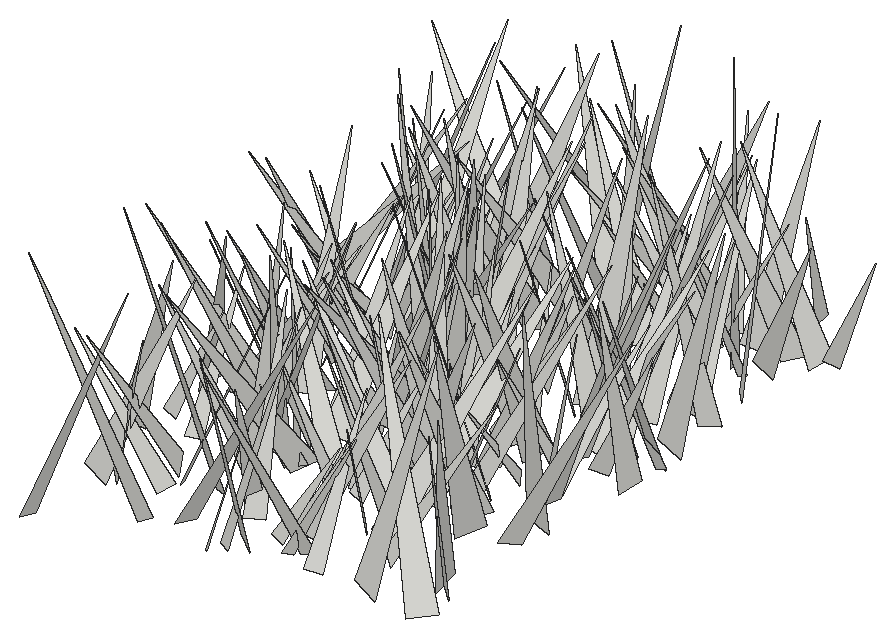
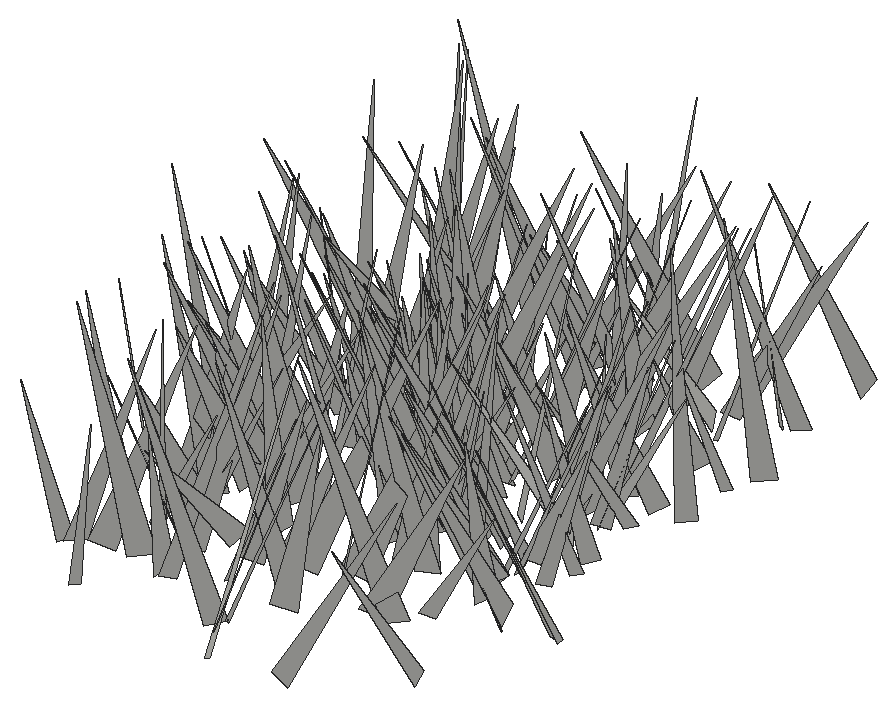
# SketchUp Ruby script. Lengths in inches.
U = 1.inch
M = Sketchup.active_model
def pt(a) = Geom::Point3d.new(a.map { |v| v * U })
def face(e, loops, mat)
  f = e.add_face(loops[0].map { |a| pt(a) })
  loops[1..].each { |l| e.add_face(l.map { |a| pt(a) }).erase! }
  f.material = f.back_material = mat if mat
  f
end
# faces: each face lists its corners as indices into pts; further lists are holes
def faces(e, pts, list, mat = nil) = list.each { |f| face(e, (f[0].is_a?(Array) ? f : [f]).map { |l| l.map { |i| pts[i] } }, mat) }
# xy, xz, yz: faces in a plane at the given z, y or x. An outline is a flat list of corners, or four numbers for a rectangle; further outlines are holes
def ring(l) = l.size == 4 ? [[l[0], l[1]], [l[2], l[1]], [l[2], l[3]], [l[0], l[3]]] : l.each_slice(2).to_a
def flat(e, list, mat, &to3) = list.each { |f| face(e, (f[0].is_a?(Array) ? f : [f]).map { |l| ring(l).map { |u, v| to3.(u, v) } }, mat) }
def xy(e, z, list, mat = nil) = flat(e, list, mat) { |x, y| [x, y, z] }
def xz(e, y, list, mat = nil) = flat(e, list, mat) { |x, z| [x, y, z] }
def yz(e, x, list, mat = nil) = flat(e, list, mat) { |y, z| [x, y, z] }
def lines(e, pts, list) = list.each { |a, b| e.add_line(pt(pts[a]), pt(pts[b])) }
# prism: a flat outline (further loops are holes) pulled along v
def prism(e, loops, v, mat = nil)
  f = face(e, loops, mat); d = Geom::Vector3d.new(v.map { |x| x * U })
  f.pushpull(f.normal.samedirection?(d) ? d.length : -d.length)
end
def box(e, o, s, mat = nil) = prism(e, [[o, [o[0] + s[0], o[1], o[2]], [o[0] + s[0], o[1] + s[1], o[2]], [o[0], o[1] + s[1], o[2]]]], [0, 0, s[2]], mat)
def at(x, y, z, deg = 0) = Geom::Transformation.translation(pt([x, y, z])) * Geom::Transformation.rotation(ORIGIN, Z_AXIS, deg.degrees)
def axes(o, x, y, z) = Geom::Transformation.new([*x, 0, *y, 0, *z, 0, *pt(o).to_a, 1])
def part(name) = M.definitions.add(name)
# library, detail: a bought-in or finely detailed component or shape, given as its bounding box
def library(name, o, s) = part(name).tap { |d| box(d.entities, o, s) }
def detail(e, o, s) = box(e.add_group.entities, o, s)
def put(e, d, t, mat = nil) = e.add_instance(d, t).tap { |i| i.material = mat if mat }
def group(e, t, mat = nil) = e.add_group.tap { |g| g.transformation = t; g.material = mat if mat }.entities
root = M.entities
c1 = part("fur_instance\#9")
p = [[0.8125,0,1.79],[0.67,-0.02,1.48],[0,-0.11,0],[0,0.11,0]]
faces(c1.entities,p,[[0,1,2,3]])
put(root,c1,axes([528.57,193.91,-21.66],[-2.74524,3.88345,0.46197],[3.73915,2.44095,1.70042],[-1.14601,-1.33847,4.4414]))
put(root,c1,axes([528.73,186.81,-21.66],[-3.23089,-3.2407,0.20186],[-3.09319,2.98531,-1.58167],[-0.98745,1.25194,4.29408]))
put(root,c1,axes([525.39,207.13,-21.66],[4.79921,1.03907,0.41248],[0.79797,-4.45725,1.94381],[-0.78297,1.82633,4.50929]))
put(root,c1,axes([522.77,199.48,-21.66],[5.32286,5.30667,0.20638],[4.93366,-4.8331,-2.97258],[1.96528,-2.23975,6.90343]))
put(root,c1,axes([526.5,195.48,-21.66],[-6.90134,-2.30385,2.57209],[-0.73953,6.60101,3.92832],[3.37291,-3.26662,6.12409]))
put(root,c1,axes([522.13,199.56,-21.66],[4.7067,5.43888,0.18038],[4.50837,-3.76361,-4.15655],[3.04771,-2.83211,5.87006]))
put(root,c1,axes([529.1875,201.72,-21.66],[-2.95637,3.32548,0.26078],[3.10336,2.61427,1.84435],[-1.22309,-1.40488,4.04936]))
put(root,c1,axes([524.52,179.79,-21.66],[2.49015,-6.48815,0.76577],[-6.33726,-2.19962,1.97082],[1.58797,1.39602,6.66429]))
put(root,c1,axes([525.36,181.79,-21.66],[0.91676,-3.52562,1.5814],[-3.59518,-0.18259,1.67709],[1.41617,1.81877,3.23385]))
put(root,c1,axes([526.02,199.09,-21.66],[6.68377,2.4417,1.0502],[1.89436,-6.36953,2.75283],[-1.86446,2.28139,6.56175]))
put(root,c1,axes([527.9,198.42,-21.66],[-5.38629,2.97439,0.98855],[2.72826,5.41671,-1.43257],[1.54299,0.80541,5.98388]))
put(root,c1,axes([528.33,195.32,-21.66],[-6.95908,-3.88864,0.42907],[-3.38575,6.42493,3.31533],[1.96017,-2.70799,7.24975]))
put(root,c1,axes([531.37,172.26,-21.66],[-3.36679,-6.63148,1.92496],[-6.20382,1.96447,-4.08298],[-3.03226,3.34389,6.21619]))
put(root,c1,axes([524.98,185.625,-21.66],[6.92696,-1.79403,0.01467],[-1.72828,-6.68834,-1.86567],[-0.48147,-1.80253,6.90801]))
put(root,c1,axes([525.2,200.62,-21.66],[3.3764,2.66955,0.1135],[2.47122,-3.05035,-1.76859],[1.01611,-1.452,3.92412]))
put(root,c1,axes([529.14,185.84,-21.66],[-7.53778,-2.79862,0.78068],[-2.32716,7.11502,3.03655],[1.73954,-2.60846,7.44512]))
put(root,c1,axes([528.0625,189.09,-21.66],[-4.13321,-3.41194,0.20507],[-3.07913,3.85633,2.10107],[1.48403,-1.5014,4.93054]))
put(root,c1,axes([531.46,203.31,-21.66],[-4.54084,5.90887,0.08971],[5.53212,4.21055,2.68494],[-2.07809,-1.7025,6.95162]))
put(root,c1,axes([528.06,188.81,-21.66],[2.83348,-4.00549,0.52306],[-3.76222,-2.8494,-1.43972],[-1.47079,-0.42795,4.69039]))
put(root,c1,axes([527.96,180.57,-21.66],[-3.50119,3.09472,0.56001],[2.74674,3.41714,-1.71109],[1.53177,0.94611,4.34831]))
put(root,c1,axes([526.14,192.05,-21.66],[2.61538,-3.98544,0.72253],[-3.93735,-2.29982,1.56655],[0.95028,1.43982,4.50221]))
put(root,c1,axes([526.34,168.91,-21.66],[6.82155,0.82248,0.97272],[0.53436,-6.65794,1.88216],[-1.15634,1.77527,6.60814]))
put(root,c1,axes([530.17,175.51,-21.66],[-4.08347,2.98679,1.40676],[3.27171,3.36098,2.36101],[-0.44252,-2.71247,4.47451]))
put(root,c1,axes([528.46,194.88,-21.66],[-4.47086,-3.62986,0.22446],[-3.11938,4.01034,2.72058],[1.8697,-1.98902,5.07572]))
put(root,c1,axes([525.89,193.55,-21.66],[1.52671,4.77623,1.67607],[4.63081,-0.61106,-2.47682],[2.04382,-2.18327,4.35989]))
put(root,c1,axes([528.67,191.63,-21.66],[3.08843,-3.08617,0.55459],[-2.71507,-3.02147,-1.69397],[-1.56857,-0.84658,4.0241]))
put(root,c1,axes([528.7,196.97,-21.66],[-6.04626,5.73242,0.3376],[5.11125,5.59588,-3.47751],[2.61721,2.31459,7.57131]))
put(root,c1,axes([528.83,195.85,-21.66],[-4.31312,-2.31019,0.44376],[-1.59331,3.55068,2.99849],[1.73068,-2.4885,3.8664]))
put(root,c1,axes([530.14,188.78,-21.66],[-0.06223,-5.95217,0.13196],[-5.73579,0.02457,-1.59678],[-1.59576,0.14382,5.73432]))
put(root,c1,axes([527.31,174.9,-21.66],[3.73633,3.15118,1.53756],[3.50493,-3.41917,-1.50964],[-0.09758,-2.15258,4.64878]))
put(root,c1,axes([530.96,211.68,-21.66],[-0.84326,-5.89202,0.02664],[-5.53518,0.78295,-2.04363],[-2.01949,0.3143,5.59022]))
put(root,c1,axes([529.37,187.77,-21.66],[-5.90287,3.96424,1.22936],[3.5461,5.92766,-2.08769],[2.15678,1.10365,6.7971]))
put(root,c1,axes([526.81,187.87,-21.66],[0.32449,4.79651,0.65441],[4.29347,0.01783,-2.25961],[2.23626,-0.73022,4.24334]))
put(root,c1,axes([529.14,177.98,-21.66],[-5.60645,-3.595,0.79099],[-2.74257,5.04084,3.47133],[2.4552,-2.57833,5.68385]))
put(root,c1,axes([528.8,193.94,-21.66],[3.99187,0.97882,1.10255],[0.50795,-3.90054,1.62373],[-1.38409,1.39155,3.77579]))
put(root,c1,axes([528.23,190.94,-21.66],[6.17595,4.1917,0.11311],[3.92557,-5.85042,2.46738],[-1.47413,1.98185,7.04448]))
put(root,c1,axes([526.33,174.45,-21.66],[1.93796,6.92662,2.2466],[6.80944,-0.90011,-3.09877],[2.58009,-2.82714,6.49087]))
put(root,c1,axes([532.58,176.99,-21.66],[-5.1387,-6.17044,1.38685],[-6.22365,4.61615,-2.52214],[-1.12419,2.64967,7.62361]))
put(root,c1,axes([528.51,196.39,-21.66],[4.2696,-0.12633,0.87704],[-0.45536,-4.01534,1.6384],[-0.76014,1.6958,3.94476]))
put(root,c1,axes([526.8,185.56,-21.66],[4.24231,-3.44067,0.07958],[-3.18347,-3.87509,2.16585],[1.3077,1.72835,5.01442]))
put(root,c1,axes([531.67,194.64,-21.66],[3.01287,6.59159,3.14785],[6.68601,-3.85992,1.68335],[-2.94198,-2.02171,7.04931]))
put(root,c1,axes([528.9,185.46,-21.66],[-0.2633,5.21725,2.01289],[5.21535,0.95622,-1.79623],[2.01778,-1.79073,4.90536]))
put(root,c1,axes([533.96,181.52,-21.66],[-0.88156,-7.55851,1.51866],[-6.98391,0.13553,-3.37952],[-3.26533,1.75074,6.81814]))
put(root,c1,axes([532.01,183.98,-21.66],[2.11114,4.26728,1.69749],[4.08085,-2.60007,1.46097],[-2.10662,-0.76029,4.53125]))
put(root,c1,axes([532.69,179.58,-21.66],[-6.28485,-0.79991,0.77187],[-0.56549,6.11624,1.73401],[0.95701,-1.63912,6.09364]))
put(root,c1,axes([532.57,184.47,-21.66],[-6.5639,-4.29471,0.69968],[-4.06333,6.50273,1.7952],[1.55674,-1.13527,7.63588]))
put(root,c1,axes([533.91,193.32,-21.66],[-6.55777,-1.69063,0.96933],[-1.94723,5.82112,-3.02077],[0.07829,3.17151,6.06115]))
put(root,c1,axes([530.46,176.52,-21.66],[5.39727,3.08007,0.18691],[2.81936,-5.07536,2.22356],[-1.25418,1.84558,5.80286]))
put(root,c1,axes([531.86,190.75,-21.66],[-4.79038,-5.44103,1.36632],[-5.2062,4.98101,1.5825],[2.08977,-0.06337,7.07448]))
put(root,c1,axes([534.72,195.49,-21.66],[-3.87014,-4.65436,0.40491],[-4.4497,3.51193,-2.16136],[-1.42379,1.67578,5.65416]))
put(root,c1,axes([532.56,179.71,-21.66],[-6.83852,1.49302,2.47832],[0.97247,7.17644,-1.63995],[2.72497,1.18576,6.80477]))
put(root,c1,axes([531.94,193.09,-21.66],[6.07778,0.82962,2.17123],[-0.33597,-5.70106,3.1188],[-2.29992,3.02515,5.28212]))
put(root,c1,axes([531.69,194.95,-21.66],[4.95008,1.27612,1.12304],[0.89586,-4.89693,1.61571],[-1.4447,1.33589,4.84988]))
put(root,c1,axes([530.04,203.27,-21.66],[-0.29437,7.39176,2.68978],[7.28817,1.26884,-2.68928],[2.95898,-2.3899,6.89148]))
put(root,c1,axes([535.32,190.75,-21.66],[0.70112,8.01126,1.73468],[7.49163,-1.33281,3.12731],[-3.32639,-1.31314,7.4089]))
put(root,c1,axes([534.32,181.81,-21.66],[4.16443,-6.48584,0.7003],[-5.50995,-3.94185,-3.74183],[-3.49241,-1.51483,6.7385]))
put(root,c1,axes([534.71,200.68,-21.66],[1.87232,-8.06563,0.81969],[-7.60481,-2.03883,-2.69107],[-2.80947,0.14362,7.83059]))
put(root,c1,axes([534.64,187.95,-21.66],[-6.99156,-3.62516,0.34789],[-3.32905,6.6672,2.57109],[1.47657,-2.13338,7.444]))
put(root,c1,axes([532.94,186.05,-21.66],[-4.70627,4.28235,1.06672],[3.70191,4.67966,-2.45399],[2.40255,1.178,5.87073]))
put(root,c1,axes([531.13,192.5625,-21.66],[8.13391,1.72844,0.70897],[1.41113,-7.75982,2.72846],[-1.22428,2.53935,7.85515]))
put(root,c1,axes([533.78,197.67,-21.66],[-6.33507,2.2676,3.27677],[3.13305,6.63723,1.4641],[2.46237,-2.61105,6.56746]))
put(root,c1,axes([535.47,205.73,-21.66],[-2.86561,6.0597,1.12131],[6.09085,2.59686,1.53195],[-0.93747,-1.65086,6.5257]))
put(root,c1,axes([533.78,203.43,-21.66],[-6.24986,-4.52728,1.84324],[-4.17742,6.50052,1.80193],[2.5383,-0.44892,7.504]))
put(root,c1,axes([534.28,200.32,-21.66],[1.52611,3.71718,0.33458],[3.41655,-1.5369,1.49113],[-1.50217,0.28087,3.73135]))
put(root,c1,axes([532.07,198.11,-21.66],[0.54119,7.40359,2.44886],[7.61955,0.0202,-1.74498],[1.65906,-2.50787,7.21533]))
put(root,c1,axes([535.94,188.21,-21.66],[-4.58905,2.11277,0.48874],[2.15665,4.32669,1.54618],[-0.22698,-1.60562,4.80963]))
put(root,c1,axes([532.86,181.7,-21.66],[-0.95701,-7.3765,1.52863],[-7.35851,1.24531,1.40248],[1.61303,1.30453,7.30491]))
put(root,c1,axes([532.6,193.82,-21.66],[4.39475,-2.24157,1.41228],[-2.61052,-4.13054,1.56743],[-0.4521,2.06082,4.67778]))
put(root,c1,axes([532.31,197.92,-21.66],[1.32188,-7.44707,0.58602],[-7.30684,-1.16527,1.67389],[1.55318,0.85612,7.37593]))
put(root,c1,axes([536.4,195.35,-21.66],[1.94153,-7.03493,2.68991],[-6.84514,-2.80689,-2.40016],[-3.14163,1.7682,6.89195]))
put(root,c1,axes([536.97,191.21,-21.66],[-4.91979,-5.33902,1.78444],[-5.59743,4.38767,-2.30455],[-0.5985,2.85253,6.88466]))
put(root,c1,axes([536.98,181.16,-21.66],[-3.95209,5.35159,0.47213],[5.26841,3.74586,1.6413],[-1.05182,-1.34553,6.44707]))
put(root,c1,axes([532.88,179.36,-21.66],[7.43701,2.08557,1.03262],[1.85087,-7.39668,1.60887],[-1.41074,1.29018,7.55449]))
put(root,c1,axes([537.23,208.98,-21.66],[-6.20853,-2.44848,0.56631],[-2.51301,6.03462,-1.45936],[-0.02325,1.56521,6.51238]))
put(root,c1,axes([533.54,185.23,-21.66],[-2.62249,6.7547,0.84995],[6.3246,2.75431,-2.37468],[2.5195,0.11678,6.84575]))
put(root,c1,axes([535.32,196.39,-21.66],[5.43527,-3.00495,4.38513],[-4.48513,-5.95873,1.47596],[-2.85354,3.64214,6.0327]))
put(root,c1,axes([535.67,175.88,-21.66],[-5.09281,3.29268,0.78292],[3.01884,5.05892,-1.63872],[1.53013,0.9783,5.83893]))
put(root,c1,axes([535.88,189.28,-21.66],[2.95419,-3.46444,1.08183],[-2.95275,-3.10527,-1.88109],[-2.11044,-0.50488,4.14621]))
put(root,c1,axes([536.98,180.97,-21.66],[-0.30638,-3.92044,1.36874],[-3.76361,-0.31774,-1.75256],[-1.75458,1.36615,3.52026]))
put(root,c1,axes([537.61,203.42,-21.66],[-2.28095,-6.51713,0.89519],[-6.46928,2.05047,-1.55597],[-1.19279,1.34151,6.72716]))
put(root,c1,axes([536.82,191.13,-21.66],[-6.72767,0.28008,1.7782],[-0.11729,6.79671,-1.51427],[1.7963,1.49276,6.56102]))
put(root,c1,axes([534.35,189.71,-21.66],[0.16131,6.95669,2.04491],[7.08472,0.28432,-1.5261],[1.54396,-2.03146,6.78915]))
put(root,c1,axes([535.84,171.74,-21.66],[2.63979,2.66437,0.28601],[2.37928,-2.51517,1.47039],[-1.23275,0.85099,3.4504]))
put(root,c1,axes([537.33,201.82,-21.66],[4.76692,-6.38187,0.99404],[-5.33821,-4.5884,-3.85875],[-3.63592,-1.6304,6.96863]))
put(root,c1,axes([536.58,189.67,-21.66],[4.8815,3.3845,2.02519],[2.72156,-5.22275,2.16824],[-2.85471,0.80828,5.53015]))
put(root,c1,axes([535.125,176.72,-21.66],[4.67947,-2.49587,0.44393],[-2.29207,-4.56374,-1.49753],[-1.08298,-1.12554,5.08765]))
put(root,c1,axes([535.3,212.25,-21.66],[-5.2335,-6.40482,0.23356],[-5.52847,4.66397,4.0186],[3.24225,-2.38569,7.22925]))
put(root,c1,axes([533.09,173.48,-21.66],[7.82793,-0.68601,0.13891],[-0.69946,-7.6099,1.83483],[0.02566,1.8399,7.64072]))
put(root,c1,axes([534.08,194.3125,-21.66],[2.99312,-6.69994,0.30324],[-6.59145,-2.87731,1.48788],[1.23852,0.87852,7.18569]))
put(root,c1,axes([534.7,188.22,-21.66],[1.84734,5.85191,0.92453],[5.8229,-1.61485,-1.41361],[1.09242,-1.28828,5.97153]))
put(root,c1,axes([534.1,196.99,-21.66],[3.571,6.90444,0.98118],[6.89309,-3.32732,-1.67343],[1.05801,-1.62595,7.59098]))
put(root,c1,axes([536.84,208.65,-21.66],[-5.34969,-3.46152,0.37635],[-2.75195,4.62606,3.43064],[2.1332,-2.713,5.36954]))
put(root,c1,axes([533.3125,192,-21.66],[6.82569,-2.14516,0.01525],[-2.06759,-6.56497,1.95405],[0.57187,1.86856,6.88284]))
put(root,c1,axes([537.81,190.9,-21.66],[-6.09704,1.94582,1.05535],[1.61207,6.02238,-1.79053],[1.51697,1.42075,6.14444]))
put(root,c1,axes([536.34,172.56,-21.66],[4.01654,5.38759,0.39242],[5.219,-3.99648,1.45013],[-1.3936,0.56102,6.56169]))
put(root,c1,axes([538.27,187.49,-21.66],[-6.12572,-2.31991,2.2614],[-2.97153,5.95041,-1.94497],[1.2907,2.68904,6.25488]))
put(root,c1,axes([536.48,204.04,-21.66],[-7.17026,0.40545,3.85637],[-0.86926,7.73252,-2.42922],[3.77894,2.54801,6.75839]))
put(root,c1,axes([537.85,188.75,-21.66],[5.96387,-5.74764,0.45925],[-4.68382,-5.21453,-4.43673],[-3.36276,-2.93042,6.99418]))
put(root,c1,axes([536.92,173.59,-21.66],[-3.51133,-6.12863,1.17286],[-5.90116,3.69891,1.66117],[2.0278,0.152,6.86513]))
put(root,c1,axes([539.97,202.88,-21.66],[-3.49983,5.63032,0.78088],[5.54982,3.18646,1.89866],[-1.22869,-1.64469,6.35172]))
put(root,c1,axes([534.82,193.79,-21.66],[4.52009,6.67395,0.30614],[6.59904,-4.40227,-1.46264],[1.04307,-1.07006,7.92676]))
put(root,c1,axes([535.83,191.75,-21.66],[2.29516,-7.21123,1.1617],[-7.23425,-2.07612,1.40519],[1.00849,1.5189,7.43607]))
put(root,c1,axes([540.28,174.66,-21.66],[-1.24481,-6.10899,0.55091],[-5.80958,0.99391,-2.10566],[-1.96776,0.93016,5.86818]))
put(root,c1,axes([538.4,185.97,-21.66],[3.46655,5.88623,0.70358],[5.62008,-3.5225,1.77941],[-1.8861,0.32244,6.59533]))
put(root,c1,axes([535.91,191.65,-21.66],[0.28527,8.21503,1.11931],[7.94931,0.04717,-2.37217],[2.35543,-1.15413,7.87026]))
put(root,c1,axes([537.84,181.71,-21.66],[4.12915,-1.39251,2.24683],[-2.1688,-4.1671,1.40312],[-1.51116,2.17563,4.12556]))
put(root,c1,axes([541.44,180.73,-21.66],[-6.06762,4.08752,0.30456],[4.00596,5.79855,1.98636],[-0.86766,-1.81261,7.04117]))
put(root,c1,axes([535.37,187.67,-21.66],[3.43501,-7.39782,1.03394],[-7.28345,-3.06455,2.27067],[1.65774,1.86463,7.83397]))
put(root,c1,axes([538.56,189.65,-21.66],[6.05789,3.57549,2.196],[3.19122,-6.43003,1.66595],[-2.72445,0.41853,6.83424]))
put(root,c1,axes([539.65,182.47,-21.66],[-5.8383,-2.13052,1.19785],[-1.77007,5.82456,1.73238],[1.68547,-1.263,5.96857]))
put(root,c1,axes([538.72,188.98,-21.66],[3.46816,-3.92613,0.03464],[-3.68547,-3.27126,-1.77763],[-1.35388,-1.15247,4.92774]))
put(root,c1,axes([535.99,187.38,-21.66],[7.97506,1.59703,0.67128],[1.71117,-7.75527,-1.87893],[-0.27022,-1.97686,7.91339]))
put(root,c1,axes([539.58,205.28,-21.66],[-4.13984,-2.04423,0.54277],[-1.65039,3.86825,1.98107],[1.32277,-1.57147,4.17043]))
put(root,c1,axes([540.73,184.64,-21.66],[-0.59735,8.07244,1.41711],[8.08686,0.34954,1.4177],[-1.33238,-1.49761,7.96939]))
put(root,c1,axes([541.54,184.15,-21.66],[1.64942,-7.33453,1.1804],[-6.83961,-1.97125,-2.69132],[-2.89974,0.47759,7.01946]))
put(root,c1,axes([538,174.9,-21.66],[1.07989,-3.22676,1.49499],[-3.22529,-0.23045,1.83235],[1.49815,1.82977,2.86716]))
put(root,c1,axes([540.63,199.62,-21.66],[-7.20595,2.28011,2.02761],[1.9171,7.42879,-1.54068],[2.37378,0.922,7.39939]))
put(root,c1,axes([538.4,180.89,-21.66],[0.79551,4.29487,0.6755],[4.10301,-0.51451,-1.56067],[1.4379,-0.90797,4.07959]))
put(root,c1,axes([541.55,179.79,-21.66],[-0.61117,-4.98438,1.28841],[-4.9544,0.21679,-1.51148],[-1.3993,1.40945,4.78884]))
put(root,c1,axes([540.75,187.05,-21.66],[-5.40299,1.91129,1.15946],[1.49374,5.34299,-1.84687],[1.66317,1.41036,5.42535]))
put(root,c1,axes([539.48,186.25,-21.66],[-1.38897,4.86037,0.26759],[4.61521,1.40338,-1.53442],[1.54748,0.17706,4.81643]))
put(root,c1,axes([537.22,209.13,-21.66],[1.67696,-6.87357,2.26471],[-6.67493,-0.57073,3.21041],[2.79647,2.7596,6.30488]))
put(root,c1,axes([543.72,185.24,-21.66],[-6.31099,-5.2237,1.0112],[-5.28027,5.95593,-2.18722],[-0.65451,2.31907,7.89505]))
put(root,c1,axes([539.35,174.03,-21.66],[3.96425,-0.56902,0.64503],[-0.79665,-3.57598,1.74151],[-0.32433,1.82859,3.60641]))
put(root,c1,axes([541.5,184.54,-21.66],[3.93699,-6.31061,2.13001],[-6.14082,-4.39732,-1.67764],[-2.57895,0.83692,7.24632]))
put(root,c1,axes([541.54,190.95,-21.66],[4.33462,-5.23656,1.50263],[-4.77333,-4.57611,-2.17783],[-2.62578,-0.3257,6.43953]))
put(root,c1,axes([538.33,196.36,-21.66],[4.58596,6.39713,1.96066],[6.63658,-4.04695,-2.31874],[0.85046,-2.91504,7.52182]))
put(root,c1,axes([544.07,196.65,-21.66],[-4.22462,-4.77942,0.40733],[-4.62488,3.91455,-2.0354],[-1.27248,1.63999,6.04544]))
put(root,c1,axes([541.57,173.4,-21.66],[-3.94545,3.07895,0.18102],[2.74281,3.63702,-2.08047],[1.41057,1.53994,4.55172]))
put(root,c1,axes([542.27,190.26,-21.66],[-4.53148,2.02632,0.31118],[1.79338,4.28391,-1.78018],[0.99329,1.50971,4.63371]))
put(root,c1,axes([538.21,177.85,-21.66],[4.07945,6.65627,1.20942],[6.56454,-3.55321,-2.58689],[1.63565,-2.3408,7.36585]))
put(root,c1,axes([543.11,203.97,-21.66],[-6.87965,3.10007,2.46286],[3.78941,6.58637,2.29475],[1.14737,-3.16466,7.18848]))
put(root,c1,axes([543.74,178.93,-21.66],[-5.8174,-1.77979,0.63377],[-1.88895,5.44209,-2.05595],[-0.03436,2.15114,5.72563]))
put(root,c1,axes([541.08,195.36,-21.66],[-4.09949,-5.26965,1.04192],[-4.89422,4.20438,2.00758],[2.21389,-0.46331,6.36747]))
put(root,c1,axes([543,194.87,-21.66],[1.40362,-5.52471,3.15038],[-5.88186,-2.35471,-1.50878],[-2.41887,2.51999,5.49692]))
put(root,c1,axes([543.6,203.23,-21.66],[-5.93019,0.58333,0.46706],[0.68124,5.75556,1.46115],[0.30714,-1.50292,5.77689]))
put(root,c1,axes([540.75,178.72,-21.66],[-2.708,-3.38854,1.07596],[-2.8715,2.88211,1.84961],[2.09627,-0.42942,3.92357]))
put(root,c1,axes([542.75,206.52,-21.66],[-5.36407,2.31527,0.60969],[2.0889,5.25672,-1.5839],[1.1699,1.22955,5.6236]))
put(root,c1,axes([541.87,201.36,-21.66],[-5.06896,3.36354,0.19703],[2.56301,4.08037,-3.71862],[2.18706,3.01393,4.81452]))
put(root,c1,axes([538.77,176.2,-21.66],[3.61026,-5.57217,1.81458],[-5.57053,-2.60139,3.09478],[1.81959,3.09184,5.87413]))
put(root,c1,axes([542.17,206.91,-21.66],[-7.59167,-1.95799,2.55179],[-0.44126,7.11339,4.14535],[3.18601,-3.68034,6.65457]))
put(root,c1,axes([539.23,185.25,-21.66],[3.81645,-5.44593,0.15233],[-5.28758,-3.65777,1.70554],[1.31259,1.09964,6.42764]))
put(root,c1,axes([540.49,184.36,-21.66],[5.57667,1.59527,0.3002],[1.43066,-5.3377,1.78788],[-0.76695,1.64269,5.51794]))
put(root,c1,axes([541.68,196.02,-21.66],[6.54564,-3.57049,3.76512],[-4.66006,-6.71077,1.73761],[-2.28219,3.46223,7.25083]))
put(root,c1,axes([540.63,190.93,-21.66],[1.73127,-4.9492,1.56465],[-4.93445,-1.0575,2.11492],[1.61056,2.08017,4.79781]))
put(root,c1,axes([541.33,182.79,-21.66],[-3.48939,6.7058,0.49493],[5.71017,3.24965,-3.77124],[3.55058,1.36403,6.55144]))
put(root,c1,axes([540.08,189.99,-21.66],[4.10846,4.74791,0.21399],[4.46685,-3.7608,-2.31765],[1.62348,-1.66782,5.83529]))
put(root,c1,axes([544.89,204.01,-21.66],[-7.31055,-2.64435,2.80127],[-3.45475,7.15889,-2.25809],[1.70424,3.16886,7.43894]))
put(root,c1,axes([542.89,183.26,-21.66],[4.06306,2.1594,0.43468],[1.91332,-3.91175,1.54848],[-1.0914,1.18135,4.33286]))
put(root,c1,axes([542.96,190.22,-21.66],[6.488,-4.94571,0.82766],[-4.48999,-6.33233,-2.64212],[-2.23271,-1.63731,7.71838]))
put(root,c1,axes([543.72,187.8,-21.66],[-3.33896,-2.6162,0.26799],[-2.1089,2.92233,2.25332],[1.57125,-1.6372,3.59384]))
put(root,c1,axes([541.6875,187.64,-21.66],[6.12264,-2.56902,1.18593],[-2.80714,-5.86992,1.77677],[-0.35534,2.10644,6.39763]))
put(root,c1,axes([545.96,203.3125,-21.66],[-1.77005,-3.87903,0.89181],[-3.77258,1.32393,-1.7292],[-1.26879,1.475,3.89741]))
put(root,c1,axes([544.72,189.77,-21.66],[-4.05266,-1.43323,0.72397],[-1.06557,3.87082,1.69814],[1.20119,-1.40176,3.94899]))
put(root,c1,axes([544.56,183.29,-21.66],[4.80853,-5.64104,1.01196],[-5.19564,-4.8483,-2.3381],[-2.41883,-0.80002,7.03396]))
put(root,c1,axes([544.95,196.4,-21.66],[-6.41092,4.00729,0.82453],[3.32918,6.00061,-3.27831],[2.37798,2.40258,6.81256]))
put(root,c1,axes([542.36,195.36,-21.66],[8.0865,0.10169,1.15451],[-0.2162,-7.86244,2.20681],[-1.13864,2.21504,7.78021]))
put(root,c1,axes([545.6,200.01,-21.66],[-5.23053,3.77379,0.03544],[3.44734,4.80229,-2.57973],[1.53577,2.07308,5.91142]))
put(root,c1,axes([542.24,178.33,-21.66],[1.49345,8.09623,0.02611],[7.76227,-1.42429,-2.34489],[2.30146,-0.44999,7.89182]))
put(root,c1,axes([546.9375,206.41,-21.66],[2.35436,-6.19743,2.05043],[-5.78585,-2.99044,-2.39512],[-3.02263,0.89697,6.18179]))
put(root,c1,axes([545.66,193.37,-21.66],[-4.8564,4.18897,0.42907],[3.70643,4.56321,-2.59917],[1.99849,1.71635,5.86314]))
put(root,c1,axes([543.1,204.3,-21.66],[3.75203,3.55416,0.24846],[3.4305,-3.50645,-1.64561],[0.96201,-1.35805,4.89916]))
put(root,c1,axes([548.77,193.06,-21.66],[-3.53185,-5.19128,1.06072],[-4.89285,2.7062,-3.04713],[-2.03336,2.50511,5.48984]))
put(root,c1,axes([542.59,185.37,-21.66],[4.68977,6.59581,0.10077],[6.41242,-4.52929,-1.96857],[1.54784,-1.22048,7.85006]))
put(root,c1,axes([544.22,195.51,-21.66],[7.47336,0.82298,1.26079],[0.38429,-7.21504,2.43175],[-1.45575,2.3203,7.11442]))
put(root,c1,axes([547.96,198.13,-21.66],[-0.65544,-6.57541,2.82853],[-6.91722,-0.14862,-1.94837],[-1.84083,2.89967,6.31422]))
put(root,c1,axes([548.9,173.23,-21.66],[-3.56857,7.17935,0.49748],[7.02506,3.35468,1.97986],[-1.56176,-1.31463,7.76903]))
put(root,c1,axes([545.5,210.47,-21.66],[4.05773,-0.76512,0.97615],[-0.40955,-3.97873,-1.41614],[-1.1707,-1.26007,3.87881]))
put(root,c1,axes([544.7,205.9,-21.66],[3.44666,-5.98968,2.82803],[-6.61551,-2.95389,1.80641],[0.33028,3.33943,6.67028]))
put(root,c1,axes([545.28,181.73,-21.66],[6.81384,-4.6319,0.82302],[-4.34734,-6.75311,-2.01405],[-1.7979,-1.22528,7.98915]))
put(root,c1,axes([544.87,191.28,-21.66],[6.92746,0.46404,1.30725],[0.06508,-6.75935,2.05449],[-1.38564,2.00246,6.63205]))
put(root,c1,axes([544.94,192.28,-21.66],[-2.23637,5.81255,0.47787],[5.16217,2.21098,-2.73477],[2.71405,0.58421,5.59536]))
put(root,c1,axes([548.34,206.8,-21.66],[-6.51837,1.52305,1.37348],[1.82295,6.39951,1.5551],[0.93967,-1.84981,6.5108]))
put(root,c1,axes([543.63,176.93,-21.66],[3.84668,4.92623,0.09388],[4.62666,-3.57049,-2.21792],[1.69428,-1.43435,5.84342]))
put(root,c1,axes([546.29,193.65,-21.66],[-1.98153,-6.18192,0.39554],[-6.00617,2.01899,1.46585],[1.5161,-0.08133,6.32408]))
put(root,c1,axes([545.38,187.98,-21.66],[4.29125,3.34973,1.68987],[3.74545,-3.97458,-1.63261],[-0.21889,-2.33948,5.19327]))
put(root,c1,axes([543.3125,195.5,-21.66],[5.8756,3.65861,0.2575],[3.32747,-5.11292,-3.2803],[1.54262,-2.90637,6.0949]))
put(root,c1,axes([547.3125,201.47,-21.66],[5.31201,5.41879,2.20999],[5.24419,-5.73235,1.45032],[-2.59727,-0.49162,7.44831]))
put(root,c1,axes([544.89,173.5,-21.66],[-0.81294,-7.33898,4.00432],[-7.82592,2.08335,2.22952],[2.94113,3.51498,7.03923]))
put(root,c1,axes([545.86,187.77,-21.66],[-0.77489,5.32124,0.74593],[4.8544,1.01638,-2.20776],[2.30365,-0.35187,4.90325]))
put(root,c1,axes([546.62,186.89,-21.66],[6.71372,1.26121,1.18447],[0.98901,-6.69183,1.51954],[-1.41968,1.3025,6.66001]))
put(root,c1,axes([545.71,198.6,-21.66],[2.64878,-6.42579,1.07864],[-6.29914,-2.22772,2.19734],[1.66585,1.79353,6.59382]))
put(root,c1,axes([547.55,184.44,-21.66],[-1.05079,-7.8114,1.55453],[-7.7743,1.34665,1.51176],[1.73053,1.30661,7.73542]))
put(root,c1,axes([546.52,190.76,-21.66],[2.75762,-4.13306,0.47465],[-3.98702,-2.46295,1.71739],[1.18791,1.32801,4.66232]))
put(root,c1,axes([548.21,193.55,-21.66],[-2.24137,-6.8028,0.2078],[-6.58087,2.22202,1.76064],[1.73594,-0.35988,6.94277]))
put(root,c1,axes([548.78,190.51,-21.66],[5.89812,-2.41371,1.85981],[-1.99813,-6.12286,-1.60962],[-2.30052,-0.87028,6.16628]))
put(root,c1,axes([546.375,204.46,-21.66],[0.60809,-6.43634,0.77652],[-5.71222,-0.16309,3.1214],[3.06594,0.97271,5.66154]))
put(root,c1,axes([547.64,176.7,-21.66],[7.1612,-0.61813,1.17268],[-0.1707,-6.81898,-2.55193],[-1.31459,-2.48182,6.71956]))
put(root,c1,axes([548.02,176.21,-21.66],[-3.37811,-5.89928,1.5704],[-5.1932,3.72048,2.80499],[3.2091,-0.18922,6.19235]))
put(root,c1,axes([547.84,194.92,-21.66],[2.12208,6.92928,3.4126],[7.54208,-1.09525,-2.46604],[1.66665,-3.86645,6.81445]))
put(root,c1,axes([547.625,182.06,-21.66],[6.83257,-2.01041,0.78824],[-2.1593,-6.33413,2.56189],[0.022,2.68032,6.64549]))
put(root,c1,axes([548.81,207.09,-21.66],[2.19638,-3.75423,0.49776],[-3.62923,-1.92217,1.51658],[1.08198,1.1735,4.07656]))
